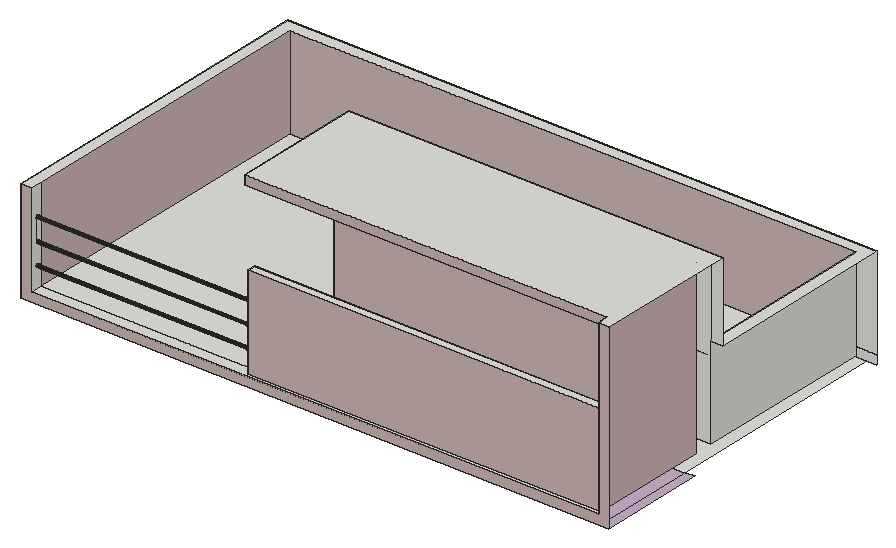
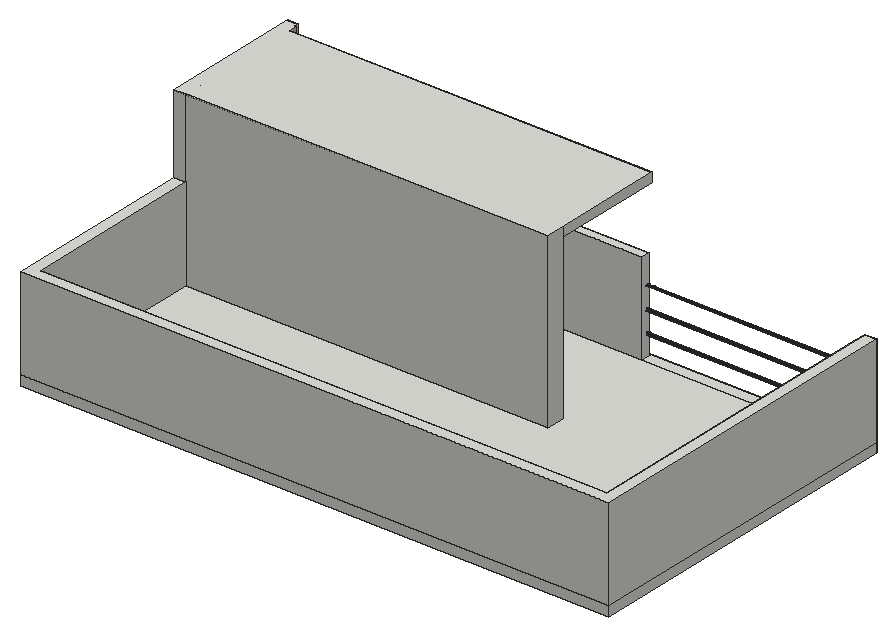
# SketchUp Ruby script. Lengths in inches.
U = 1.inch
M = Sketchup.active_model
def pt(a) = Geom::Point3d.new(a.map { |v| v * U })
def face(e, loops, mat)
  f = e.add_face(loops[0].map { |a| pt(a) })
  loops[1..].each { |l| e.add_face(l.map { |a| pt(a) }).erase! }
  f.material = f.back_material = mat if mat
  f
end
# faces: each face lists its corners as indices into pts; further lists are holes
def faces(e, pts, list, mat = nil) = list.each { |f| face(e, (f[0].is_a?(Array) ? f : [f]).map { |l| l.map { |i| pts[i] } }, mat) }
# xy, xz, yz: faces in a plane at the given z, y or x. An outline is a flat list of corners, or four numbers for a rectangle; further outlines are holes
def ring(l) = l.size == 4 ? [[l[0], l[1]], [l[2], l[1]], [l[2], l[3]], [l[0], l[3]]] : l.each_slice(2).to_a
def flat(e, list, mat, &to3) = list.each { |f| face(e, (f[0].is_a?(Array) ? f : [f]).map { |l| ring(l).map { |u, v| to3.(u, v) } }, mat) }
def xy(e, z, list, mat = nil) = flat(e, list, mat) { |x, y| [x, y, z] }
def xz(e, y, list, mat = nil) = flat(e, list, mat) { |x, z| [x, y, z] }
def yz(e, x, list, mat = nil) = flat(e, list, mat) { |y, z| [x, y, z] }
def lines(e, pts, list) = list.each { |a, b| e.add_line(pt(pts[a]), pt(pts[b])) }
# prism: a flat outline (further loops are holes) pulled along v
def prism(e, loops, v, mat = nil)
  f = face(e, loops, mat); d = Geom::Vector3d.new(v.map { |x| x * U })
  f.pushpull(f.normal.samedirection?(d) ? d.length : -d.length)
end
def box(e, o, s, mat = nil) = prism(e, [[o, [o[0] + s[0], o[1], o[2]], [o[0] + s[0], o[1] + s[1], o[2]], [o[0], o[1] + s[1], o[2]]]], [0, 0, s[2]], mat)
def at(x, y, z, deg = 0) = Geom::Transformation.translation(pt([x, y, z])) * Geom::Transformation.rotation(ORIGIN, Z_AXIS, deg.degrees)
def axes(o, x, y, z) = Geom::Transformation.new([*x, 0, *y, 0, *z, 0, *pt(o).to_a, 1])
def part(name) = M.definitions.add(name)
# library, detail: a bought-in or finely detailed component or shape, given as its bounding box
def library(name, o, s) = part(name).tap { |d| box(d.entities, o, s) }
def detail(e, o, s) = box(e.add_group.entities, o, s)
def put(e, d, t, mat = nil) = e.add_instance(d, t).tap { |i| i.material = mat if mat }
def group(e, t, mat = nil) = e.add_group.tap { |g| g.transformation = t; g.material = mat if mat }.entities
root = M.entities
M.materials.add("[0007_MistyRose]").color = [206, 184, 182]
M.materials.add("[0118_Thistle]").color = [198, 175, 198]
M.materials.add("[Translucent Glass Blue]").color = [100, 149, 237]
M.materials["[Translucent Glass Blue]"].alpha = 0.5
M.materials.add("[Wood Cherry Original]").color = [152, 86, 42]
xy(root,1443.99,[[984.34,288,1028.68,289],[1028.68,288,1073.02,289],[1081.02,288,1125.36,289],[1125.36,288,1169.7,289]])
xy(root,1536,[[0,12,24,876],[24,288,1500,876]])
xy(root,1536,[[24,12,1500,288],[1500,12,1524,288]],"[0118_Thistle]")
xy(root,1560,[[30,12,581.91,42],[581.91,12,1496.42,21],[30,42,1494,42,1494,330,556.9375,330,556.9375,378,1494,378,1494,846,30,846]])
xy(root,1800,[[0,12,30,12,30,846,1494,846,1494,378,1524,378,1524,876,0,876],[581.91,21,1494,42]])
xy(root,1980,[[556.9375,42,1494,330]],"[0007_MistyRose]")
xy(root,2004,[[1496.42,12,1524,12,1524,378,556.9375,378,556.9375,42,1494,42,1494,21,1496.42,21]])
xz(root,12,[[0,1536,1524,1536,1524,2004,1496.42,2004,1496.42,1560,30,1560,30,1800,0,1800]],"[0007_MistyRose]")
xz(root,21,[[581.91,1560,1496.42,1560,1496.42,2004,1494,2004,1494,1800,581.91,1800]],"[0007_MistyRose]")
xz(root,42,[[581.91,1560,1494,1800]])
xz(root,42,[[556.9375,1980,1494,2004]],"[0007_MistyRose]")
xz(root,289,[[984.34,1338.08,1028.68,1443.99],[1028.68,1338.08,1073.02,1443.99],[1081.02,1338.08,1125.36,1443.99],[1125.36,1338.08,1169.7,1443.99]],"[Translucent Glass Blue]")
xz(root,330,[[556.9375,1560,1494,1980]],"[0007_MistyRose]")
xz(root,378,[[556.9375,1560,1494,2004],[1494,1800,1524,2004]])
xz(root,846,[[30,1560,1494,1800]],"[0007_MistyRose]")
xz(root,876,[[0,1536,1524,1560],[0,1560,1524,1800]])
yz(root,0,[[12,1536,876,1560],[12,1560,876,1800]])
yz(root,30,[[[12,1560,27,1560,27,1612.34,26.22,1612.4375,25.5,1612.74,24.88,1613.22,24.4,1613.84,24.1,1614.5625,24,1615.34,24.1,1616.11,24.4,1616.84,24.88,1617.46,25.5,1617.94,26.22,1618.23,27,1618.34,27,1667.67,26.22,1667.78,25.5,1668.08,24.88,1668.55,24.4,1669.17,24.1,1669.9,24,1670.67,24.1,1671.45,24.4,1672.17,24.88,1672.8,25.5,1673.27,26.22,1673.57,27,1673.67,27.78,1673.57,28.5,1673.27,29.12,1672.8,29.6,1672.17,29.9,1671.45,30,1670.67,29.9,1669.9,29.6,1669.17,29.12,1668.55,28.5,1668.08,27.78,1667.78,27,1667.67,27,1618.34,27.78,1618.23,28.5,1617.94,29.12,1617.46,29.6,1616.84,29.9,1616.11,30,1615.34,29.9,1614.5625,29.6,1613.84,29.12,1613.22,28.5,1612.74,27.78,1612.4375,27,1612.34,27,1560,42,1560,42,1800,12,1800],[27,1725,26.22,1725.1,25.5,1725.4,24.88,1725.88,24.4,1726.5,24.1,1727.22,24,1728,24.1,1728.78,24.4,1729.5,24.88,1730.12,25.5,1730.6,26.22,1730.9,27,1731,27.78,1730.9,28.5,1730.6,29.12,1730.12,29.6,1729.5,29.9,1728.78,30,1728,29.9,1727.22,29.6,1726.5,29.12,1725.88,28.5,1725.4,27.78,1725.1]]])
yz(root,30,[[42,1560,846,1800]],"[0007_MistyRose]")
yz(root,556.9375,[[330,1560,378,2004],[42,1980,330,2004]])
yz(root,581.91,[[[21,1560,42,1800],[27,1725,27.78,1725.1,28.5,1725.4,29.12,1725.88,29.6,1726.5,29.9,1727.22,30,1728,29.9,1728.78,29.6,1729.5,29.12,1730.12,28.5,1730.6,27.78,1730.9,27,1731,26.22,1730.9,25.5,1730.6,24.88,1730.12,24.4,1729.5,24.1,1728.78,24,1728,24.1,1727.22,24.4,1726.5,24.88,1725.88,25.5,1725.4,26.22,1725.1],[27,1667.67,27.78,1667.78,28.5,1668.08,29.12,1668.55,29.6,1669.17,29.9,1669.9,30,1670.67,29.9,1671.45,29.6,1672.17,29.12,1672.8,28.5,1673.27,27.78,1673.57,27,1673.67,26.22,1673.57,25.5,1673.27,24.88,1672.8,24.4,1672.17,24.1,1671.45,24,1670.67,24.1,1669.9,24.4,1669.17,24.88,1668.55,25.5,1668.08,26.22,1667.78],[27,1612.34,27.78,1612.4375,28.5,1612.74,29.12,1613.22,29.6,1613.84,29.9,1614.5625,30,1615.34,29.9,1616.11,29.6,1616.84,29.12,1617.46,28.5,1617.94,27.78,1618.23,27,1618.34,26.22,1618.23,25.5,1617.94,24.88,1617.46,24.4,1616.84,24.1,1616.11,24,1615.34,24.1,1614.5625,24.4,1613.84,24.88,1613.22,25.5,1612.74,26.22,1612.4375]],[27,1612.34,27.78,1612.4375,28.5,1612.74,29.12,1613.22,29.6,1613.84,29.9,1614.5625,30,1615.34,29.9,1616.11,29.6,1616.84,29.12,1617.46,28.5,1617.94,27.78,1618.23,27,1618.34,26.22,1618.23,25.5,1617.94,24.88,1617.46,24.4,1616.84,24.1,1616.11,24,1615.34,24.1,1614.5625,24.4,1613.84,24.88,1613.22,25.5,1612.74,26.22,1612.4375],[27,1667.67,27.78,1667.78,28.5,1668.08,29.12,1668.55,29.6,1669.17,29.9,1669.9,30,1670.67,29.9,1671.45,29.6,1672.17,29.12,1672.8,28.5,1673.27,27.78,1673.57,27,1673.67,26.22,1673.57,25.5,1673.27,24.88,1672.8,24.4,1672.17,24.1,1671.45,24,1670.67,24.1,1669.9,24.4,1669.17,24.88,1668.55,25.5,1668.08,26.22,1667.78],[27,1725,27.78,1725.1,28.5,1725.4,29.12,1725.88,29.6,1726.5,29.9,1727.22,30,1728,29.9,1728.78,29.6,1729.5,29.12,1730.12,28.5,1730.6,27.78,1730.9,27,1731,26.22,1730.9,25.5,1730.6,24.88,1730.12,24.4,1729.5,24.1,1728.78,24,1728,24.1,1727.22,24.4,1726.5,24.88,1725.88,25.5,1725.4,26.22,1725.1]])
yz(root,984.34,[[288,1338.08,289,1443.99]])
yz(root,1073.02,[[288,1338.08,289,1443.99]])
yz(root,1081.02,[[288,1338.08,289,1443.99]])
yz(root,1169.7,[[288,1338.08,289,1443.99]])
yz(root,1494,[[378,1560,846,1800]])
yz(root,1494,[[42,1560,330,1980],[21,1800,42,2004]],"[0007_MistyRose]")
yz(root,1496.42,[[12,1560,21,2004]],"[0007_MistyRose]")
p = [[581.91,27,1612.34],[581.91,26.22,1612.4375],[30,26.22,1612.4375],[30,27,1612.34],[581.91,27.78,1612.4375],[30,27.78,1612.4375],
  [581.91,25.5,1612.74],[30,25.5,1612.74],[581.91,28.5,1612.74],[30,28.5,1612.74],[581.91,24.88,1613.22],[30,24.88,1613.22],
  [581.91,29.12,1613.22],[30,29.12,1613.22],[581.91,24.4,1613.84],[30,24.4,1613.84],[581.91,29.6,1613.84],[30,29.6,1613.84],
  [581.91,24.1,1614.5625],[30,24.1,1614.5625],[581.91,29.9,1614.5625],[30,29.9,1614.5625],[581.91,24,1615.34],[30,24,1615.34],
  [581.91,30,1615.34],[30,30,1615.34],[581.91,24.1,1616.11],[30,24.1,1616.11],[581.91,29.9,1616.11],[30,29.9,1616.11],
  [581.91,24.4,1616.84],[30,24.4,1616.84],[581.91,29.6,1616.84],[30,29.6,1616.84],[581.91,24.88,1617.46],[30,24.88,1617.46],
  [581.91,29.12,1617.46],[30,29.12,1617.46],[581.91,25.5,1617.94],[30,25.5,1617.94],[581.91,28.5,1617.94],[30,28.5,1617.94],
  [581.91,26.22,1618.23],[30,26.22,1618.23],[581.91,27.78,1618.23],[30,27.78,1618.23],[581.91,27,1618.34],[30,27,1618.34],
  [581.91,27,1667.67],[581.91,26.22,1667.78],[30,26.22,1667.78],[30,27,1667.67],[581.91,27.78,1667.78],[30,27.78,1667.78],
  [581.91,25.5,1668.08],[30,25.5,1668.08],[581.91,28.5,1668.08],[30,28.5,1668.08],[581.91,24.88,1668.55],[30,24.88,1668.55],
  [581.91,29.12,1668.55],[30,29.12,1668.55],[581.91,24.4,1669.17],[30,24.4,1669.17],[581.91,29.6,1669.17],[30,29.6,1669.17],
  [581.91,24.1,1669.9],[30,24.1,1669.9],[581.91,29.9,1669.9],[30,29.9,1669.9],[581.91,24,1670.67],[30,24,1670.67],
  [581.91,30,1670.67],[30,30,1670.67],[581.91,24.1,1671.45],[30,24.1,1671.45],[581.91,29.9,1671.45],[30,29.9,1671.45],
  [581.91,24.4,1672.17],[30,24.4,1672.17],[581.91,29.6,1672.17],[30,29.6,1672.17],[581.91,24.88,1672.8],[30,24.88,1672.8],
  [581.91,29.12,1672.8],[30,29.12,1672.8],[581.91,25.5,1673.27],[30,25.5,1673.27],[581.91,28.5,1673.27],[30,28.5,1673.27],
  [581.91,26.22,1673.57],[30,26.22,1673.57],[581.91,27.78,1673.57],[30,27.78,1673.57],[581.91,27,1673.67],[30,27,1673.67],
  [567.75,26.22,1725.1],[30,26.22,1725.1],[30,27,1725],[567.75,27,1725],[581.91,27,1725],[581.91,26.22,1725.1],
  [30,27.78,1725.1],[567.75,27.78,1725.1],[581.91,27.78,1725.1],[567.75,25.5,1725.4],[30,25.5,1725.4],[581.91,25.5,1725.4],
  [30,28.5,1725.4],[567.75,28.5,1725.4],[581.91,28.5,1725.4],[567.75,24.88,1725.88],[30,24.88,1725.88],[581.91,24.88,1725.88],
  [30,29.12,1725.88],[567.75,29.12,1725.88],[581.91,29.12,1725.88],[567.75,24.4,1726.5],[30,24.4,1726.5],[581.91,24.4,1726.5],
  [30,29.6,1726.5],[567.75,29.6,1726.5],[581.91,29.6,1726.5],[567.75,24.1,1727.22],[30,24.1,1727.22],[581.91,24.1,1727.22],
  [30,29.9,1727.22],[567.75,29.9,1727.22],[581.91,29.9,1727.22],[567.75,24,1728],[30,24,1728],[581.91,24,1728],
  [30,30,1728],[567.75,30,1728],[581.91,30,1728],[567.75,24.1,1728.78],[30,24.1,1728.78],[581.91,24.1,1728.78],
  [30,29.9,1728.78],[567.75,29.9,1728.78],[581.91,29.9,1728.78],[567.75,24.4,1729.5],[30,24.4,1729.5],[581.91,24.4,1729.5],
  [30,29.6,1729.5],[567.75,29.6,1729.5],[581.91,29.6,1729.5],[567.75,24.88,1730.12],[30,24.88,1730.12],[581.91,24.88,1730.12],
  [30,29.12,1730.12],[567.75,29.12,1730.12],[581.91,29.12,1730.12],[567.75,25.5,1730.6],[30,25.5,1730.6],[581.91,25.5,1730.6],
  [30,28.5,1730.6],[567.75,28.5,1730.6],[581.91,28.5,1730.6],[567.75,26.22,1730.9],[30,26.22,1730.9],[581.91,26.22,1730.9],
  [30,27.78,1730.9],[567.75,27.78,1730.9],[581.91,27.78,1730.9],[567.75,27,1731],[30,27,1731],[581.91,27,1731],
  [1524,330,1800],[1494,330,1800],[1494,330,1980],[1494,330,2004],[30,27,1728],[567.75,27,1728],
  [581.91,27,1728],[30,27,1670.67],[581.91,27,1670.67],[30,27,1615.34],[581.91,27,1615.34]]
faces(root,p,[[0,1,2,3],[4,0,3,5],[1,6,7,2],[8,4,5,9],[6,10,11,7],[12,8,9,13],[10,14,15,11],[16,12,13,17],
  [14,18,19,15],[20,16,17,21],[18,22,23,19],[24,20,21,25],[22,26,27,23],[28,24,25,29],[26,30,31,27],[32,28,29,33],
  [30,34,35,31],[36,32,33,37],[34,38,39,35],[40,36,37,41],[38,42,43,39],[44,40,41,45],[42,46,47,43],[46,44,45,47],
  [48,49,50,51],[52,48,51,53],[49,54,55,50],[56,52,53,57],[54,58,59,55],[60,56,57,61],[58,62,63,59],[64,60,61,65],
  [62,66,67,63],[68,64,65,69],[66,70,71,67],[72,68,69,73],[70,74,75,71],[76,72,73,77],[74,78,79,75],[80,76,77,81],
  [78,82,83,79],[84,80,81,85],[82,86,87,83],[88,84,85,89],[86,90,91,87],[92,88,89,93],[90,94,95,91],[94,92,93,95],
  [96,97,98,99,100,101],[99,98,102,103,104,100],[105,106,97,96,101,107],[103,102,108,109,110,104],[111,112,106,105,107,113],[109,108,114,115,116,110],[117,118,112,111,113,119],[115,114,120,121,122,116],
  [123,124,118,117,119,125],[121,120,126,127,128,122],[129,130,124,123,125,131],[127,126,132,133,134,128],[135,136,130,129,131,137],[133,132,138,139,140,134],[141,142,136,135,137,143],[139,138,144,145,146,140],
  [147,148,142,141,143,149],[145,144,150,151,152,146],[153,154,148,147,149,155],[151,150,156,157,158,152],[159,160,154,153,155,161],[157,156,162,163,164,158],[165,166,160,159,161,167],[163,162,166,165,167,164]],"[Wood Cherry Original]")
lines(root,p,[[168,169],[170,171],[172,173],[173,174],[175,95],[175,176],[177,47],[177,178],[98,172],[95,98],[51,175],[3,177]])
